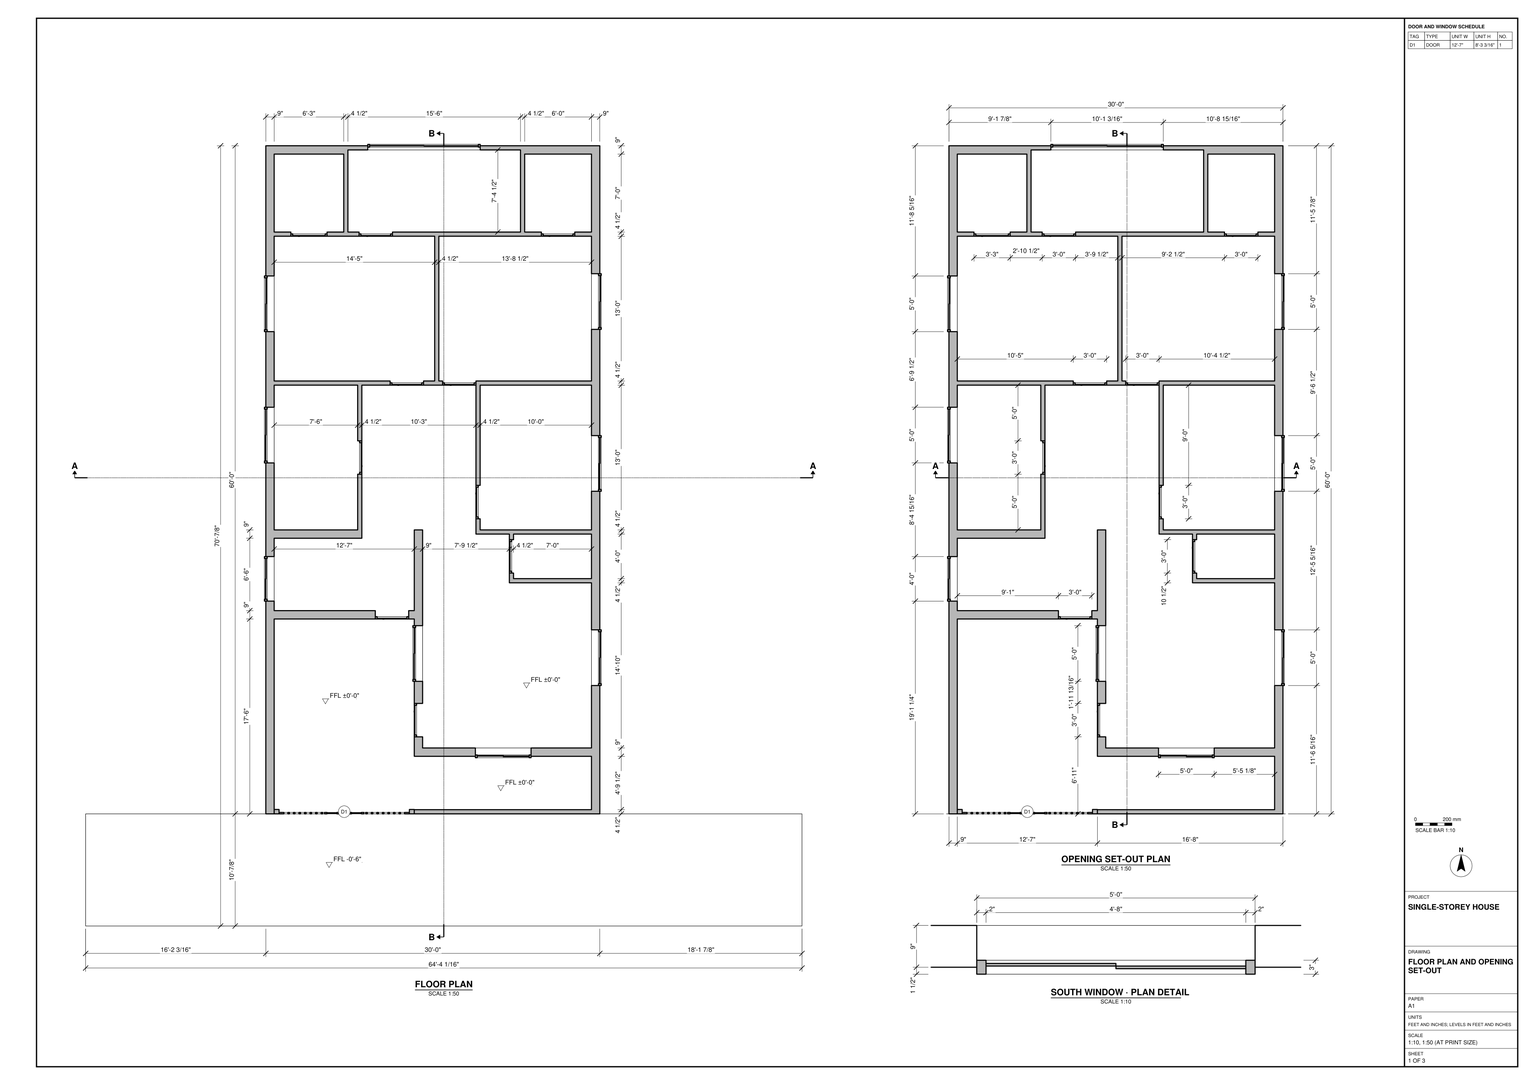
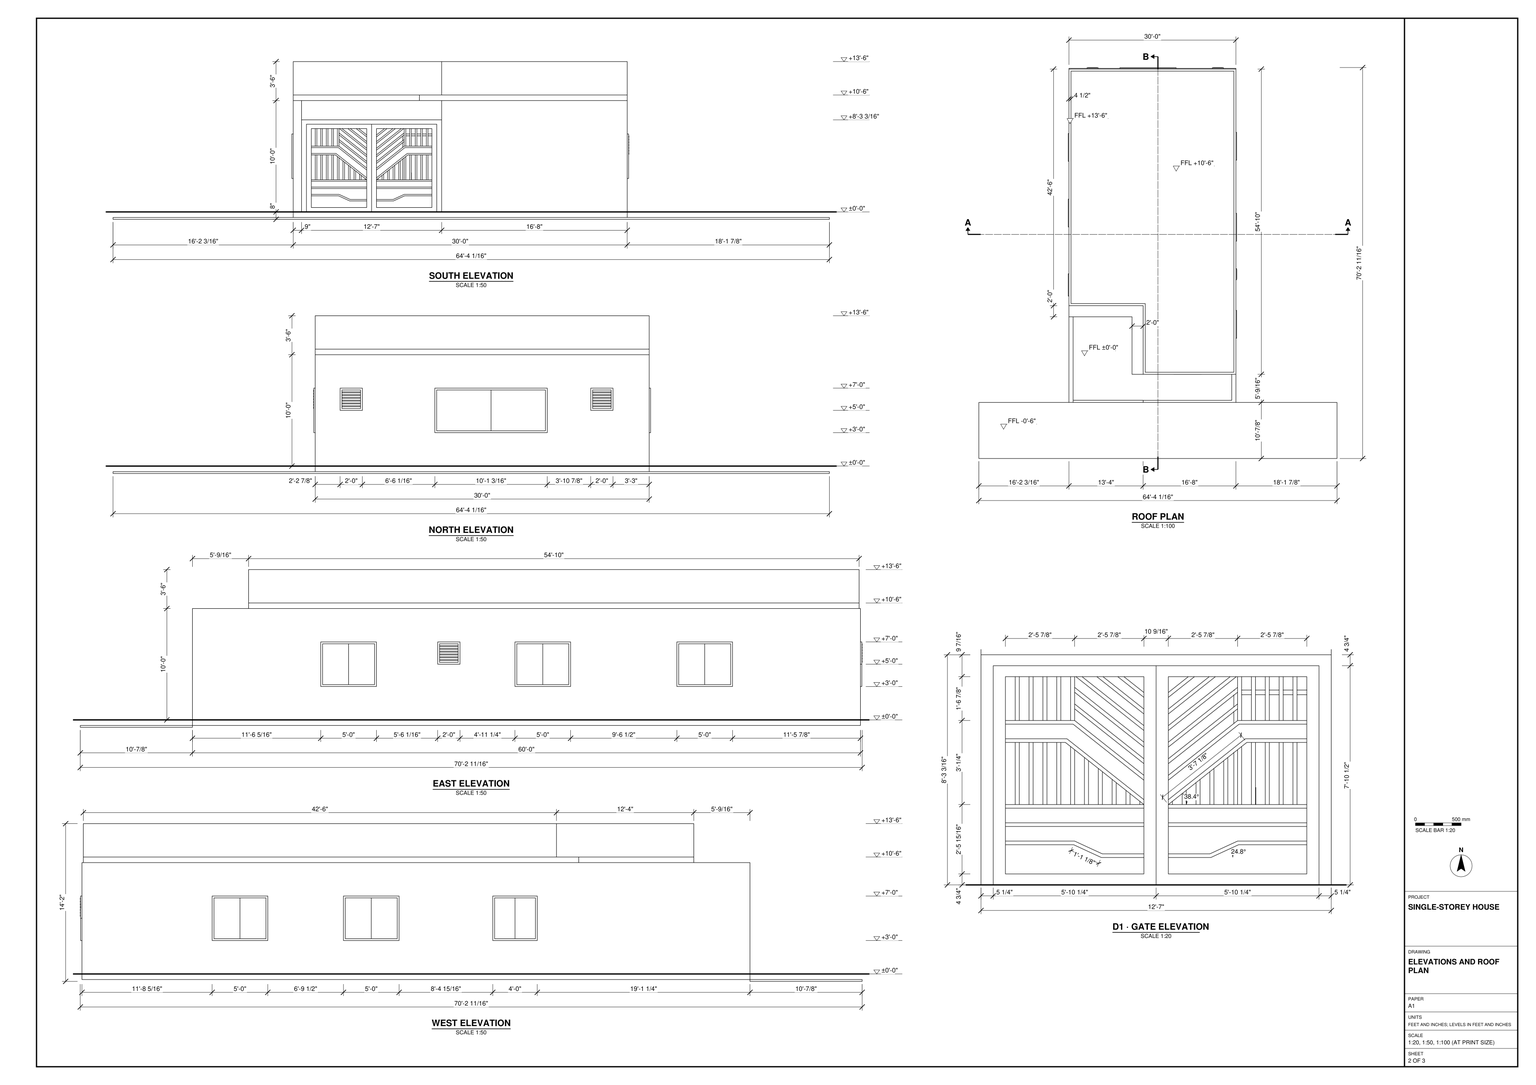
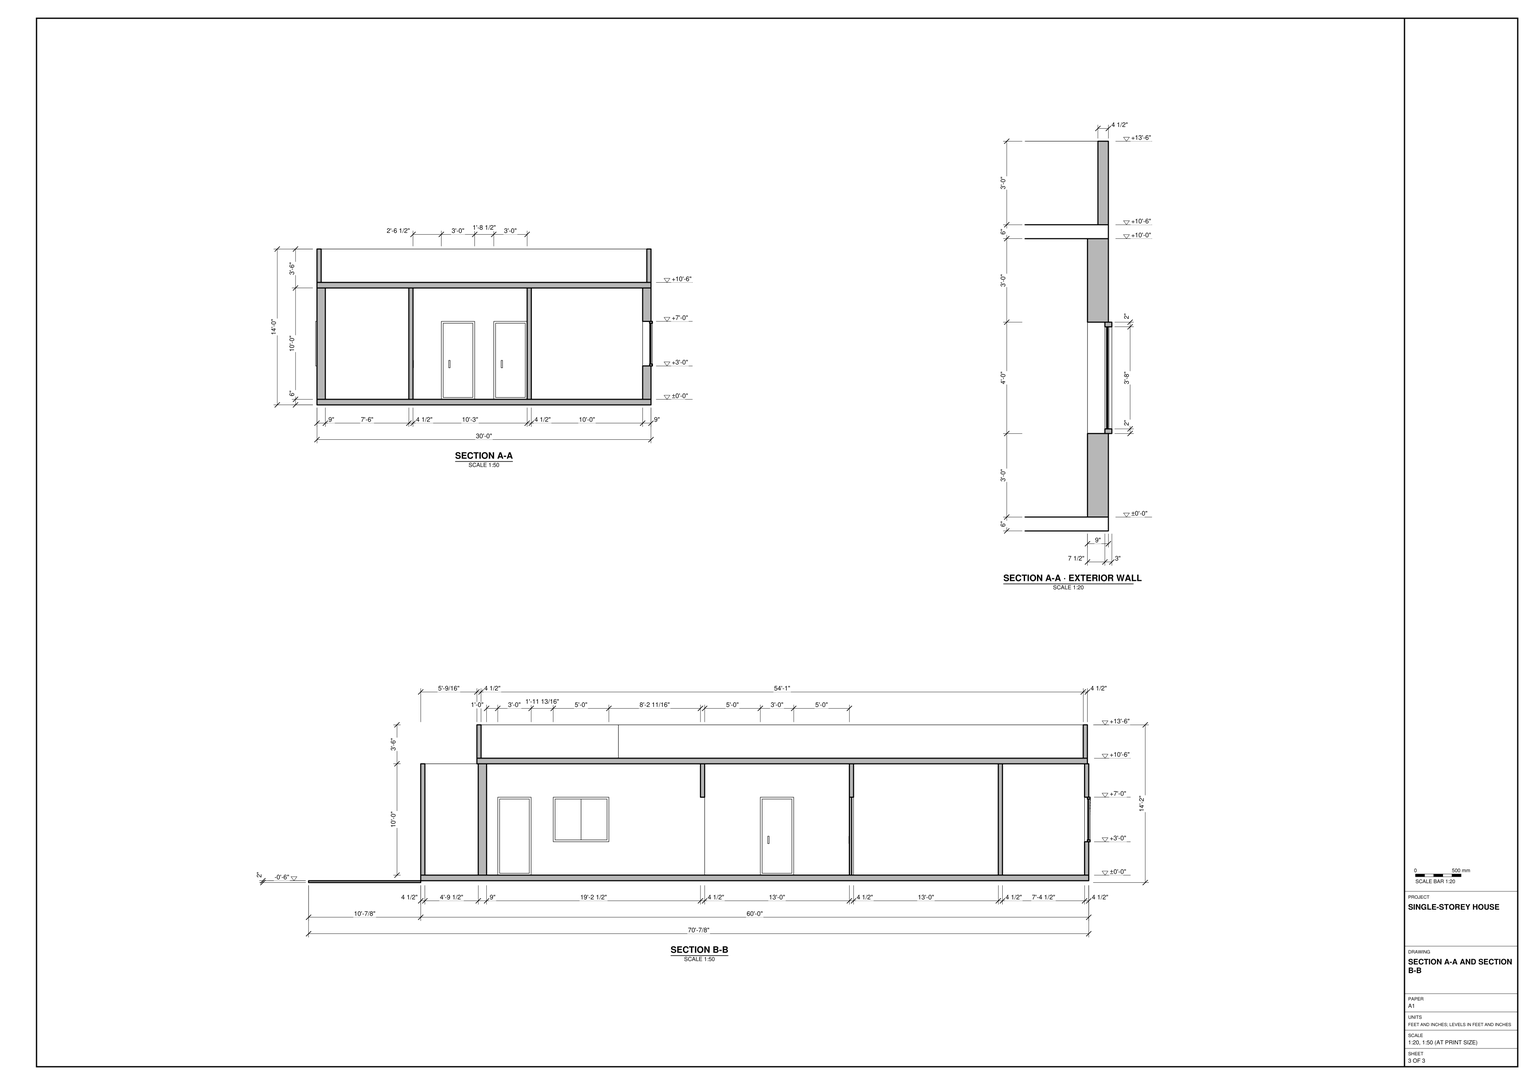
Build the house in SketchUp from task_files/diagram_01.pdf. Work in feet and inches. Including the frontage strip, the model measures 64'-4 1/16" east–west, 70'-2 11/16" north–south and 14'-2" high. Use ±0'-0" as the finished floor level of the single storey. Set the strip outside the south gate 6" below the finished floor and extend it beyond both sides of the house as drawn.

Use the floor plan to lay out the 30'-0" by 60'-0" enclosure, the open front court and the rooms behind it. Distinguish the 9" exterior walls from the 4 1/2" partitions, retaining the thicker wall sections marked on the plan. Use the opening set-out plan for doorway and window positions and the elevations for sill and head heights. Model the south gate with two framed leaves and mirrored diagonal infill. Follow the roof plan around the court recess and use the sections to set the floor slab, flat roof slab and parapet heights.

Keep the walls, slabs, roof and opening units separately editable as groups or components. Keep each furniture or joinery piece separate if shown, and use components for repeated parts. Decor and loose items may be any suitable library components. Save one SketchUp model as output_files/single_storey_house_with_a_gated_front_court.skp.

# SketchUp Ruby script. Lengths in inches.
U = 1.inch
M = Sketchup.active_model
def pt(a) = Geom::Point3d.new(a.map { |v| v * U })
def face(e, loops, mat)
  f = e.add_face(loops[0].map { |a| pt(a) })
  loops[1..].each { |l| e.add_face(l.map { |a| pt(a) }).erase! }
  f.material = f.back_material = mat if mat
  f
end
# faces: each face lists its corners as indices into pts; further lists are holes
def faces(e, pts, list, mat = nil) = list.each { |f| face(e, (f[0].is_a?(Array) ? f : [f]).map { |l| l.map { |i| pts[i] } }, mat) }
# xy, xz, yz: faces in a plane at the given z, y or x. An outline is a flat list of corners, or four numbers for a rectangle; further outlines are holes
def ring(l) = l.size == 4 ? [[l[0], l[1]], [l[2], l[1]], [l[2], l[3]], [l[0], l[3]]] : l.each_slice(2).to_a
def flat(e, list, mat, &to3) = list.each { |f| face(e, (f[0].is_a?(Array) ? f : [f]).map { |l| ring(l).map { |u, v| to3.(u, v) } }, mat) }
def xy(e, z, list, mat = nil) = flat(e, list, mat) { |x, y| [x, y, z] }
def xz(e, y, list, mat = nil) = flat(e, list, mat) { |x, z| [x, y, z] }
def yz(e, x, list, mat = nil) = flat(e, list, mat) { |y, z| [x, y, z] }
def lines(e, pts, list) = list.each { |a, b| e.add_line(pt(pts[a]), pt(pts[b])) }
# prism: a flat outline (further loops are holes) pulled along v
def prism(e, loops, v, mat = nil)
  f = face(e, loops, mat); d = Geom::Vector3d.new(v.map { |x| x * U })
  f.pushpull(f.normal.samedirection?(d) ? d.length : -d.length)
end
def box(e, o, s, mat = nil) = prism(e, [[o, [o[0] + s[0], o[1], o[2]], [o[0] + s[0], o[1] + s[1], o[2]], [o[0], o[1] + s[1], o[2]]]], [0, 0, s[2]], mat)
def at(x, y, z, deg = 0) = Geom::Transformation.translation(pt([x, y, z])) * Geom::Transformation.rotation(ORIGIN, Z_AXIS, deg.degrees)
def axes(o, x, y, z) = Geom::Transformation.new([*x, 0, *y, 0, *z, 0, *pt(o).to_a, 1])
def part(name) = M.definitions.add(name)
# library, detail: a bought-in or finely detailed component or shape, given as its bounding box
def library(name, o, s) = part(name).tap { |d| box(d.entities, o, s) }
def detail(e, o, s) = box(e.add_group.entities, o, s)
def put(e, d, t, mat = nil) = e.add_instance(d, t).tap { |i| i.material = mat if mat }
def group(e, t, mat = nil) = e.add_group.tap { |g| g.transformation = t; g.material = mat if mat }.entities
root = M.entities
M.materials.add("Asphalt A02 100cm").color = [81, 81, 83]
M.materials.add("Brown Tiles 240cm").color = [175, 145, 136]
M.materials.add("Glass Smoked Distorted 001").color = [38, 38, 38]
M.materials["Glass Smoked Distorted 001"].alpha = 0.1
M.materials.add("Granite Black Pearl 150cm").color = [48, 48, 48]
M.materials.add("Iron Blurry").color = [53, 53, 53]
M.materials.add("Porcelain Dusk Blue Glossy Rough 001").color = [122, 143, 157]
M.materials.add("Porcelain Poised Taupe Glossy Rough 001").color = [140, 135, 132]
M.materials.add("Two Color Maple Panels 300cm").color = [56, 46, 41]
c1 = library("gate 119k",[0,1.18,0],[135.43,4.73,99.21])
c2 = part("Group\#5")
box(c2.entities,[0,0,0],[0.31,28,44])
c3 = part("Group\#7")
box(c3.entities,[0,0,0],[0.31,28,44])
c4 = part("Group\#9")
box(c4.entities,[0,0,0],[20,0.31,2])
c5 = part("Group\#11")
box(c5.entities,[0,0,0],[20,0.31,2])
c6 = part("Group\#13")
box(c6.entities,[-0.31,0,0],[0.31,28,44])
c7 = part("Group\#15")
box(c7.entities,[-0.5,0,0],[0.5,28,44])
c8 = part("Group\#17")
box(c8.entities,[0,0,0],[0.31,20,2])
c9 = part("Group\#19")
box(c9.entities,[-0.31,0,0],[0.31,28,44])
c10 = part("Group\#21")
box(c10.entities,[0,0,0],[28,0.56,44])
c11 = part("Group\#23")
box(c11.entities,[0,0,0],[0.31,28,44])
c12 = part("Group\#55")
box(c12.entities,[0,-0.31,0],[58.59,0.31,44])
put(root,c1,axes([203.1875,119.69,14.43],[1.11494,0,0],[0,1,0],[0,0,1]))
g1 = group(root,at(194.1875,120.875,14.43))
xy(g1,0,[[[9,0,160,0,160,4.5,351,4.5,351,62,160,62,160,83,169,83,169,71,351,71,351,249,262.5,249,262.5,259.5,267,259.5,267,253.5,351,253.5,351,301.5,267,301.5,267,295.5,262.5,295.5,262.5,301.5,226.5,301.5,226.5,318,231,318,231,306,351,306,351,462,231,462,231,354,226.5,354,226.5,466.5,351,466.5,351,622.5,333,622.5,333,627,351,627,351,711,279,711,279,627,297,627,297,622.5,186.5,622.5,186.5,466.5,190.5,466.5,190.5,462,170,462,170,466.5,182,466.5,182,622.5,136.5,622.5,136.5,627,274.5,627,274.5,715.5,88.5,715.5,88.5,627,100.5,627,100.5,622.5,66,622.5,66,627,84,627,84,711,9,711,9,627,27,627,27,622.5,9,622.5,9,466.5,134,466.5,134,462,103.5,462,103.5,402,99,402,99,462,9,462,9,306,99,306,99,366,103.5,366,103.5,297,9,297,9,219,118,219,118,210,9,210],[160,119,160,210,154,210,154,219,160,219,160,306,169,306,169,119]]],"Granite Black Pearl 150cm")
xy(g1,36,[[225.875,62,285.875,71],[351,138.3125,360,198.3125],[160,142.8125,169,202.8125],[0,229.25,9,277.25],[351,347.625,360,407.625],
  [0,378.1875,9,438.1875],[0,519.6875,9,579.6875],[351,522.125,360,582.125],[109.875,715.5,231.0625,720]],"Porcelain Dusk Blue Glossy Rough 001")
xy(g1,60,[[351,264.375,360,288.375],[39,711,63,720],[309.125,711,333.125,720]],"Porcelain Dusk Blue Glossy Rough 001")
xy(g1,84,[[225.875,62,285.875,71],[160,83,169,119],[351,138.3125,360,198.3125],[160,142.8125,169,202.8125],[118,210,154,219],
  [0,229.25,9,277.25],[262.5,259.5,267,295.5],[351,264.375,360,288.375],[103.5,301.5,160,306],[169,301.5,226.5,306],
  [226.5,318,231,354],[351,347.625,360,407.625],[99,366,103.5,402],[0,378.1875,9,438.1875],[134,462,170,466.5],
  [190.5,462,226.5,466.5],[0,519.6875,9,579.6875],[351,522.125,360,582.125],[27,622.5,66,627],[100.5,622.5,136.5,627],
  [297,622.5,333,627],[39,711,63,720],[309.125,711,333.125,720],[109.875,715.5,231.0625,720]],"Porcelain Dusk Blue Glossy Rough 001")
xy(g1,120,[[[0,0,9,0,9,210,160,210,160,62,351,62,351,4.5,160,4.5,160,0,360,0,360,720,0,720],[169,71,169,301.5,262.5,301.5,262.5,249,351,249,351,71],[9,466.5,182,622.5],[186.5,466.5,351,622.5],[103.5,306,226.5,462],[231,306,351,462],[88.5,627,274.5,715.5],[9,306,99,462],[9,219,9,297,103.5,297,103.5,301.5,160,301.5,160,219],[9,627,84,711],[279,627,351,711],[267,253.5,351,301.5]]],"Porcelain Dusk Blue Glossy Rough 001")
xz(g1,0,[[0,0,9,120],[160,0,360,120]],"Porcelain Dusk Blue Glossy Rough 001")
xz(g1,4.5,[[160,0,351,120]],"Porcelain Dusk Blue Glossy Rough 001")
xz(g1,62,[[[160,0,351,120],[225.875,36,285.875,84]]],"Porcelain Dusk Blue Glossy Rough 001")
xz(g1,71,[[[169,0,351,120],[225.875,36,285.875,84]]],"Porcelain Dusk Blue Glossy Rough 001")
xz(g1,83,[[160,0,169,84]],"Porcelain Dusk Blue Glossy Rough 001")
xz(g1,119,[[160,0,169,84]],"Porcelain Dusk Blue Glossy Rough 001")
xz(g1,138.3125,[[351,36,360,84]],"Porcelain Dusk Blue Glossy Rough 001")
xz(g1,142.8125,[[160,36,169,84]],"Porcelain Dusk Blue Glossy Rough 001")
xz(g1,198.3125,[[351,36,360,84]],"Porcelain Dusk Blue Glossy Rough 001")
xz(g1,202.8125,[[160,36,169,84]],"Porcelain Dusk Blue Glossy Rough 001")
xz(g1,210,[[9,0,118,0,118,84,154,84,154,0,160,0,160,120,9,120]],"Porcelain Dusk Blue Glossy Rough 001")
xz(g1,219,[[9,0,9,120,160,120,160,0,154,0,154,84,118,84,118,0]],"Porcelain Dusk Blue Glossy Rough 001")
xz(g1,229.25,[[0,36,9,84]],"Porcelain Dusk Blue Glossy Rough 001")
xz(g1,249,[[262.5,0,351,120]],"Porcelain Dusk Blue Glossy Rough 001")
xz(g1,253.5,[[267,0,351,120]],"Porcelain Dusk Blue Glossy Rough 001")
xz(g1,259.5,[[262.5,0,267,84]],"Porcelain Dusk Blue Glossy Rough 001")
xz(g1,264.375,[[351,60,360,84]],"Porcelain Dusk Blue Glossy Rough 001")
xz(g1,277.25,[[0,36,9,84]],"Porcelain Dusk Blue Glossy Rough 001")
xz(g1,288.375,[[351,60,360,84]],"Porcelain Dusk Blue Glossy Rough 001")
xz(g1,295.5,[[262.5,0,267,84]],"Porcelain Dusk Blue Glossy Rough 001")
xz(g1,297,[[9,0,103.5,120]],"Porcelain Dusk Blue Glossy Rough 001")
xz(g1,301.5,[[226.5,0,262.5,0,262.5,120,169,120,169,84,226.5,84],[267,0,351,120],[103.5,84,160,120]],"Porcelain Dusk Blue Glossy Rough 001")
xz(g1,306,[[9,0,99,120],[160,0,160,84,103.5,84,103.5,120,226.5,120,226.5,84,169,84,169,0],[231,0,351,120]],"Porcelain Dusk Blue Glossy Rough 001")
xz(g1,318,[[226.5,0,231,84]],"Porcelain Dusk Blue Glossy Rough 001")
xz(g1,347.625,[[351,36,360,84]],"Porcelain Dusk Blue Glossy Rough 001")
xz(g1,354,[[226.5,0,231,84]],"Porcelain Dusk Blue Glossy Rough 001")
xz(g1,366,[[99,0,103.5,84]],"Porcelain Dusk Blue Glossy Rough 001")
xz(g1,378.1875,[[0,36,9,84]],"Porcelain Dusk Blue Glossy Rough 001")
xz(g1,402,[[99,0,103.5,84]],"Porcelain Dusk Blue Glossy Rough 001")
xz(g1,407.625,[[351,36,360,84]],"Porcelain Dusk Blue Glossy Rough 001")
xz(g1,438.1875,[[0,36,9,84]],"Porcelain Dusk Blue Glossy Rough 001")
xz(g1,462,[[9,0,99,120],[103.5,0,134,0,134,84,170,84,170,0,190.5,0,190.5,84,226.5,84,226.5,120,103.5,120],[231,0,351,120]],"Porcelain Dusk Blue Glossy Rough 001")
xz(g1,466.5,[[9,0,9,120,182,120,182,0,170,0,170,84,134,84,134,0],[186.5,0,186.5,120,351,120,351,0,226.5,0,226.5,84,190.5,84,190.5,0]],"Porcelain Dusk Blue Glossy Rough 001")
xz(g1,519.6875,[[0,36,9,84]],"Porcelain Dusk Blue Glossy Rough 001")
xz(g1,522.125,[[351,36,360,84]],"Porcelain Dusk Blue Glossy Rough 001")
xz(g1,579.6875,[[0,36,9,84]],"Porcelain Dusk Blue Glossy Rough 001")
xz(g1,582.125,[[351,36,360,84]],"Porcelain Dusk Blue Glossy Rough 001")
xz(g1,622.5,[[9,0,27,0,27,84,66,84,66,0,100.5,0,100.5,84,136.5,84,136.5,0,182,0,182,120,9,120],[186.5,0,297,0,297,84,333,84,333,0,351,0,351,120,186.5,120]],"Porcelain Dusk Blue Glossy Rough 001")
xz(g1,627,[[9,0,9,120,84,120,84,0,66,0,66,84,27,84,27,0],[88.5,0,88.5,120,274.5,120,274.5,0,136.5,0,136.5,84,100.5,84,100.5,0],[279,0,279,120,351,120,351,0,333,0,333,84,297,84,297,0]],"Porcelain Dusk Blue Glossy Rough 001")
xz(g1,711,[[[9,0,84,120],[39,60,63,84]],[[279,0,351,120],[309.125,60,333.125,84]]],"Porcelain Dusk Blue Glossy Rough 001")
xz(g1,715.5,[[[88.5,0,274.5,120],[109.875,36,231.0625,84]]],"Porcelain Dusk Blue Glossy Rough 001")
xz(g1,720,[[[0,0,360,120],[109.875,36,231.0625,84],[309.125,60,333.125,84],[39,60,63,84]]],"Porcelain Dusk Blue Glossy Rough 001")
yz(g1,0,[[[0,0,720,120],[519.6875,36,579.6875,84],[378.1875,36,438.1875,84],[229.25,36,277.25,84]]],"Porcelain Dusk Blue Glossy Rough 001")
yz(g1,9,[[0,0,210,120],[[219,0,297,120],[229.25,36,277.25,84]],[[306,0,462,120],[378.1875,36,438.1875,84]],[[466.5,0,622.5,120],[519.6875,36,579.6875,84]],[627,0,711,120]],"Porcelain Dusk Blue Glossy Rough 001")
yz(g1,27,[[622.5,0,627,84]],"Porcelain Dusk Blue Glossy Rough 001")
yz(g1,39,[[711,60,720,84]],"Porcelain Dusk Blue Glossy Rough 001")
yz(g1,63,[[711,60,720,84]],"Porcelain Dusk Blue Glossy Rough 001")
yz(g1,66,[[622.5,0,627,84]],"Porcelain Dusk Blue Glossy Rough 001")
yz(g1,84,[[627,0,711,120]],"Porcelain Dusk Blue Glossy Rough 001")
yz(g1,88.5,[[627,0,715.5,120]],"Porcelain Dusk Blue Glossy Rough 001")
yz(g1,99,[[306,0,306,120,462,120,462,0,402,0,402,84,366,84,366,0]],"Porcelain Dusk Blue Glossy Rough 001")
yz(g1,100.5,[[622.5,0,627,84]],"Porcelain Dusk Blue Glossy Rough 001")
yz(g1,103.5,[[297,0,366,0,366,84,402,84,402,0,462,0,462,120,306,120,306,84,301.5,84,301.5,120,297,120]],"Porcelain Dusk Blue Glossy Rough 001")
yz(g1,109.875,[[715.5,36,720,84]],"Porcelain Dusk Blue Glossy Rough 001")
yz(g1,118,[[210,0,219,84]],"Porcelain Dusk Blue Glossy Rough 001")
yz(g1,134,[[462,0,466.5,84]],"Porcelain Dusk Blue Glossy Rough 001")
yz(g1,136.5,[[622.5,0,627,84]],"Porcelain Dusk Blue Glossy Rough 001")
yz(g1,154,[[210,0,219,84]],"Porcelain Dusk Blue Glossy Rough 001")
yz(g1,160,[[0,0,4.5,120],[[62,0,62,120,210,120,210,0,119,0,119,84,83,84,83,0],[142.8125,36,202.8125,84]],[219,0,219,120,301.5,120,301.5,84,306,84,306,0]],"Porcelain Dusk Blue Glossy Rough 001")
yz(g1,169,[[[71,0,83,0,83,84,119,84,119,0,306,0,306,84,301.5,84,301.5,120,71,120],[142.8125,36,202.8125,84]]],"Porcelain Dusk Blue Glossy Rough 001")
yz(g1,170,[[462,0,466.5,84]],"Porcelain Dusk Blue Glossy Rough 001")
yz(g1,182,[[466.5,0,622.5,120]],"Porcelain Dusk Blue Glossy Rough 001")
yz(g1,186.5,[[466.5,0,622.5,120]],"Porcelain Dusk Blue Glossy Rough 001")
yz(g1,190.5,[[462,0,466.5,84]],"Porcelain Dusk Blue Glossy Rough 001")
yz(g1,225.875,[[62,36,71,84]],"Porcelain Dusk Blue Glossy Rough 001")
yz(g1,226.5,[[301.5,0,301.5,84,306,84,306,120,462,120,462,84,466.5,84,466.5,0,354,0,354,84,318,84,318,0]],"Porcelain Dusk Blue Glossy Rough 001")
yz(g1,231,[[306,0,318,0,318,84,354,84,354,0,462,0,462,120,306,120]],"Porcelain Dusk Blue Glossy Rough 001")
yz(g1,231.0625,[[715.5,36,720,84]],"Porcelain Dusk Blue Glossy Rough 001")
yz(g1,262.5,[[249,0,249,120,301.5,120,301.5,0,295.5,0,295.5,84,259.5,84,259.5,0]],"Porcelain Dusk Blue Glossy Rough 001")
yz(g1,267,[[253.5,0,259.5,0,259.5,84,295.5,84,295.5,0,301.5,0,301.5,120,253.5,120]],"Porcelain Dusk Blue Glossy Rough 001")
yz(g1,274.5,[[627,0,715.5,120]],"Porcelain Dusk Blue Glossy Rough 001")
yz(g1,279,[[627,0,711,120]],"Porcelain Dusk Blue Glossy Rough 001")
yz(g1,285.875,[[62,36,71,84]],"Porcelain Dusk Blue Glossy Rough 001")
yz(g1,297,[[622.5,0,627,84]],"Porcelain Dusk Blue Glossy Rough 001")
yz(g1,309.125,[[711,60,720,84]],"Porcelain Dusk Blue Glossy Rough 001")
yz(g1,333,[[622.5,0,627,84]],"Porcelain Dusk Blue Glossy Rough 001")
yz(g1,333.125,[[711,60,720,84]],"Porcelain Dusk Blue Glossy Rough 001")
yz(g1,351,[[4.5,0,62,120],[[71,0,249,120],[138.3125,36,198.3125,84]],[[253.5,0,301.5,120],[264.375,60,288.375,84]],[[306,0,462,120],[347.625,36,407.625,84]],[[466.5,0,622.5,120],[522.125,36,582.125,84]],
  [627,0,711,120]],"Porcelain Dusk Blue Glossy Rough 001")
yz(g1,360,[[[0,0,720,120],[138.3125,36,198.3125,84],[347.625,36,407.625,84],[522.125,36,582.125,84],[264.375,60,288.375,84]]],"Porcelain Dusk Blue Glossy Rough 001")
g2 = group(g1,at(0,229.25,36))
prism(g2,[[[-1.5,48,0],[-1.5,0,0],[-1.5,0,48],[-1.5,48,48]],[[-1.5,2,46],[-1.5,2,2],[-1.5,46,2],[-1.5,46,46]]],[3,0,0],"Iron Blurry")
g3 = group(g2,at(-0.0625,24,2),"Glass Smoked Distorted 001")
box(g3,[0,0,0],[0.31,22,44],"Glass Smoked Distorted 001")
g4 = group(g2,at(-0.38,2,2),"Glass Smoked Distorted 001")
box(g4,[0,0,0],[0.31,22,44],"Glass Smoked Distorted 001")
g5 = group(g1,at(0,378.1875,36))
prism(g5,[[[-1.5,60,0],[-1.5,0,0],[-1.5,0,48],[-1.5,60,48]],[[-1.5,58,46],[-1.5,2,46],[-1.5,2,2],[-1.5,58,2]]],[3,0,0],"Iron Blurry")
put(g5,c2,at(-0.125,30,2),"Glass Smoked Distorted 001")
put(g5,c2,at(-0.44,2,2),"Glass Smoked Distorted 001")
g6 = group(g1,at(0,519.6875,36))
prism(g6,[[[-1.5,60,0],[-1.5,0,0],[-1.5,0,48],[-1.5,60,48]],[[-1.5,58,46],[-1.5,2,46],[-1.5,2,2],[-1.5,58,2]]],[3,0,0],"Iron Blurry")
put(g6,c3,at(0.1875,30,2),"Glass Smoked Distorted 001")
put(g6,c3,at(-0.13,2,2),"Glass Smoked Distorted 001")
g7 = group(g1,at(39,720,60))
prism(g7,[[[24,1.5,0],[0,1.5,0],[0,1.5,24],[24,1.5,24]],[[2,1.5,2],[22,1.5,2],[22,1.5,22],[2,1.5,22]]],[0,-3,0],"Iron Blurry")
put(g7,c4,at(2,1.5,20),"Glass Smoked Distorted 001")
put(g7,c4,at(2,1.45,17),"Glass Smoked Distorted 001")
put(g7,c4,at(2,1.4,14),"Glass Smoked Distorted 001")
put(g7,c4,at(2,1.34,11),"Glass Smoked Distorted 001")
put(g7,c4,at(2,1.29,8),"Glass Smoked Distorted 001")
put(g7,c4,at(2,1.24,5),"Glass Smoked Distorted 001")
put(g7,c4,at(2,1.19,2),"Glass Smoked Distorted 001")
g8 = group(g1,at(309.125,720,60))
prism(g8,[[[24,1.5,0],[0,1.5,0],[0,1.5,24],[24,1.5,24]],[[2,1.5,22],[2,1.5,2],[22,1.5,2],[22,1.5,22]]],[0,-3,0],"Iron Blurry")
put(g8,c5,at(2,1.5,20),"Glass Smoked Distorted 001")
put(g8,c5,at(2,1.5,17),"Glass Smoked Distorted 001")
put(g8,c5,at(2,1.5,14),"Glass Smoked Distorted 001")
put(g8,c5,at(2,1.5,11),"Glass Smoked Distorted 001")
put(g8,c5,at(2,1.5,8),"Glass Smoked Distorted 001")
put(g8,c5,at(2,1.5,5),"Glass Smoked Distorted 001")
put(g8,c5,at(2,1.5,2),"Glass Smoked Distorted 001")
g9 = group(g1,at(360,522.125,36))
prism(g9,[[[1.5,0,0],[1.5,60,0],[1.5,60,48],[1.5,0,48]],[[1.5,2,46],[1.5,58,46],[1.5,58,2],[1.5,2,2]]],[-3,0,0],"Iron Blurry")
put(g9,c6,at(0.1875,2,2),"Glass Smoked Distorted 001")
put(g9,c6,at(0.5,30,2),"Glass Smoked Distorted 001")
g10 = group(g1,at(360,347.625,36))
prism(g10,[[[1.5,0,0],[1.5,60,0],[1.5,60,48],[1.5,0,48]],[[1.5,58,2],[1.5,2,2],[1.5,2,46],[1.5,58,46]]],[-3,0,0],"Iron Blurry")
put(g10,c7,at(-0.25,2,2),"Glass Smoked Distorted 001")
put(g10,c7,at(0.25,30,2),"Glass Smoked Distorted 001")
g11 = group(g1,at(360,264.375,60))
prism(g11,[[[1.5,0,0],[1.5,24,0],[1.5,24,24],[1.5,0,24]],[[1.5,22,22],[1.5,22,2],[1.5,2,2],[1.5,2,22]]],[-3,0,0],"Iron Blurry")
put(g11,c8,at(1.5,2,20),"Glass Smoked Distorted 001")
put(g11,c8,at(1.5,2,17),"Glass Smoked Distorted 001")
put(g11,c8,at(1.5,2,14),"Glass Smoked Distorted 001")
put(g11,c8,at(1.5,2,11),"Glass Smoked Distorted 001")
put(g11,c8,at(1.5,2,8),"Glass Smoked Distorted 001")
put(g11,c8,at(1.5,2,5),"Glass Smoked Distorted 001")
put(g11,c8,at(1.5,2,2),"Glass Smoked Distorted 001")
g12 = group(g1,at(360,138.3125,36))
prism(g12,[[[1.5,0,0],[1.5,60,0],[1.5,60,48],[1.5,0,48]],[[1.5,58,46],[1.5,58,2],[1.5,2,2],[1.5,2,46]]],[-3,0,0],"Iron Blurry")
put(g12,c9,at(0.125,2,2),"Glass Smoked Distorted 001")
put(g12,c9,at(0.44,30,2),"Glass Smoked Distorted 001")
g13 = group(g1,at(225.875,62,36))
prism(g13,[[[0,-1.5,0],[60,-1.5,0],[60,-1.5,48],[0,-1.5,48]],[[2,-1.5,46],[58,-1.5,46],[58,-1.5,2],[2,-1.5,2]]],[0,3,0],"Iron Blurry")
put(g13,c10,at(2,0.25,2),"Glass Smoked Distorted 001")
put(g13,c10,at(30,-0.31,2),"Glass Smoked Distorted 001")
g14 = group(g1,at(160,142.8125,36))
prism(g14,[[[-1.5,0,0],[-1.5,0,48],[-1.5,60,48],[-1.5,60,0]],[[-1.5,2,46],[-1.5,2,2],[-1.5,58,2],[-1.5,58,46]]],[3,0,0],"Iron Blurry")
put(g14,c11,at(0,30,2),"Glass Smoked Distorted 001")
put(g14,c11,at(-0.31,2,2),"Glass Smoked Distorted 001")
g15 = group(g1,at(118,210,0))
prism(g15,[[[36,0,0],[36,0,84],[0,0,84],[0,0,0]],[[2,0,82],[34,0,82],[34,0,2],[2,0,2]]],[0,2.5,0],"Iron Blurry")
g16 = group(g15,at(2,0,2))
box(g16,[0,0,0],[32,0.71,80],"Two Color Maple Panels 300cm")
g17 = group(g16,at(6,0,32))
box(g17,[0,-0.5,0],[1.5,0.5,8],"Iron Blurry")
g18 = group(g1,at(160,83,0))
prism(g18,[[[0,36,0],[0,0,0],[0,0,84],[0,36,84]],[[0,34,2],[0,34,82],[0,2,82],[0,2,2]]],[2.5,0,0],"Iron Blurry")
g19 = group(g18,at(0,2,2))
box(g19,[0,0,0],[0.71,32,80],"Two Color Maple Panels 300cm")
g20 = group(g19,at(0,26,32))
box(g20,[-0.5,-1.5,0],[0.5,1.5,8],"Iron Blurry")
g21 = group(g1,at(262.5,259.5,0))
prism(g21,[[[0,36,0],[0,0,0],[0,0,84],[0,36,84]],[[0,34,2],[0,34,82],[0,2,82],[0,2,2]]],[2.5,0,0],"Iron Blurry")
g22 = group(g21,at(0,2,2))
box(g22,[0,0,0],[0.71,32,80],"Two Color Maple Panels 300cm")
g23 = group(g22,at(0,26,32),"Iron Blurry")
box(g23,[-0.5,-1.5,0],[0.5,1.5,8])
g24 = group(g1,at(226.5,318,0))
prism(g24,[[[0,0,0],[0,0,84],[0,36,84],[0,36,0]],[[0,2,2],[0,34,2],[0,34,82],[0,2,82]]],[2.5,0,0],"Iron Blurry")
g25 = group(g24,at(0,2,2))
box(g25,[0,0,0],[0.71,32,80],"Two Color Maple Panels 300cm")
g26 = group(g25,at(0,26,32),"Iron Blurry")
box(g26,[-0.5,-1.5,0],[0.5,1.5,8])
g27 = group(g1,at(103.5,366,0))
prism(g27,[[[0,36,0],[0,36,84],[0,0,84],[0,0,0]],[[0,34,82],[0,34,2],[0,2,2],[0,2,82]]],[-2.5,0,0],"Iron Blurry")
g28 = group(g27,at(0,2,2))
box(g28,[-0.71,0,0],[0.71,32,80],"Two Color Maple Panels 300cm")
g29 = group(g28,at(0,6,32))
box(g29,[0,0,0],[0.5,1.5,8],"Iron Blurry")
g30 = group(g1,at(134,462,0))
prism(g30,[[[36,0,0],[36,0,84],[0,0,84],[0,0,0]],[[2,0,82],[34,0,82],[34,0,2],[2,0,2]]],[0,2.5,0],"Iron Blurry")
g31 = group(g30,at(2,0,2))
box(g31,[0,0,0],[32,0.71,80],"Two Color Maple Panels 300cm")
g32 = group(g31,at(6,0,32),"Iron Blurry")
box(g32,[0,-0.5,0],[1.5,0.5,8])
g33 = group(g1,at(27,622.5,0))
prism(g33,[[[39,0,0],[39,0,84],[0,0,84],[0,0,0]],[[37,0,82],[37,0,2],[2,0,2],[2,0,82]]],[0,2.5,0],"Iron Blurry")
g34 = group(g33,at(2,0,2))
box(g34,[0,0,0],[35,0.71,80],"Two Color Maple Panels 300cm")
g35 = group(g34,at(6,0,32),"Iron Blurry")
box(g35,[0,-0.5,0],[1.5,0.5,8])
g36 = group(g1,at(100.5,622.5,0))
prism(g36,[[[36,0,0],[36,0,84],[0,0,84],[0,0,0]],[[34,0,2],[2,0,2],[2,0,82],[34,0,82]]],[0,2.5,0],"Iron Blurry")
g37 = group(g36,at(2,0,2))
xy(g37,0,[[0,0,32,0.71]])
xy(g37,80,[[0,0,32,0.71]])
xz(g37,0,[[0,0,32,80]],"Two Color Maple Panels 300cm")
xz(g37,0.71,[[0,0,32,80]])
yz(g37,0,[[0,0,0.71,80]])
yz(g37,32,[[0,0,0.71,80]])
g38 = group(g37,at(6,0,32),"Iron Blurry")
box(g38,[0,-0.5,0],[1.5,0.5,8],"Iron Blurry")
g39 = group(g1,at(297,622.5,0))
prism(g39,[[[36,0,0],[36,0,84],[0,0,84],[0,0,0]],[[2,0,2],[2,0,82],[34,0,82],[34,0,2]]],[0,2.5,0],"Iron Blurry")
g40 = group(g39,at(2,0,2))
box(g40,[0,0,0],[32,0.71,80],"Two Color Maple Panels 300cm")
g41 = group(g40,at(6,0,32),"Iron Blurry")
box(g41,[0,-0.5,0],[1.5,0.5,8])
g42 = group(g1,at(190.5,462,0))
prism(g42,[[[36,0,0],[36,0,84],[0,0,84],[0,0,0]],[[34,0,82],[34,0,2],[2,0,2],[2,0,82]]],[0,2.5,0],"Iron Blurry")
g43 = group(g42,at(2,0,2))
xy(g43,0,[[0,0,32,0.71]])
xy(g43,80,[[0,0,32,0.71]])
xz(g43,0,[[0,0,32,80]],"Two Color Maple Panels 300cm")
xz(g43,0.71,[[0,0,32,80]])
yz(g43,0,[[0,0,0.71,80]])
yz(g43,32,[[0,0,0.71,80]])
g44 = group(g43,at(6,0,32),"Iron Blurry")
box(g44,[0,-0.5,0],[1.5,0.5,8])
g45 = group(g1,at(109.875,720,36))
prism(g45,[[[121.1875,1.5,0],[0,1.5,0],[0,1.5,48],[121.1875,1.5,48]],[[2,1.5,46],[2,1.5,2],[119.1875,1.5,2],[119.1875,1.5,46]]],[0,-3,0],"Iron Blurry")
put(g45,c12,at(60.59,-0.0625,2),"Glass Smoked Distorted 001")
put(g45,c12,at(2,0.25,2),"Glass Smoked Distorted 001")
g46 = group(root,at(194.1875,120.875,14.43))
box(g46,[0,0,-6],[360,720,6],"Granite Black Pearl 150cm")
g47 = group(root,at(194.1875,181.42,134.43))
xy(g47,6,[[136,0,160,0,160,148,0,148,0,124,136,124]],"Brown Tiles 240cm")
g48 = group(g47,at(0,-62,0))
xy(g48,0,[[136,62,136,186,0,186,0,720,360,720,360,62]])
xy(g48,6,[[136,62,360,62,360,720,0,720,0,186,136,186]],"Brown Tiles 240cm")
xz(g48,62,[[136,0,360,6]])
xz(g48,186,[[0,0,136,6]])
xz(g48,720,[[0,0,360,6]])
yz(g48,0,[[186,0,720,6]])
yz(g48,136,[[62,0,186,6]])
yz(g48,360,[[62,0,720,6]])
g49 = group(g48,at(0,62,6),"Porcelain Poised Taupe Glossy Rough 001")
prism(g49,[[[160,148,0],[0,148,0],[0,658,0],[360,658,0],[360,0,0],[160,0,0]],[[4.5,653.5,0],[4.5,152.5,0],[164.5,152.5,0],[164.5,4.5,0],[355.5,4.5,0],[355.5,653.5,0]]],[0,0,36],"Porcelain Poised Taupe Glossy Rough 001")
g50 = group(root,at(194.1875,0,8.43),"Asphalt A02 100cm")
box(g50,[-194.1875,0,-2],[772.0625,120.875,2],"Asphalt A02 100cm")
